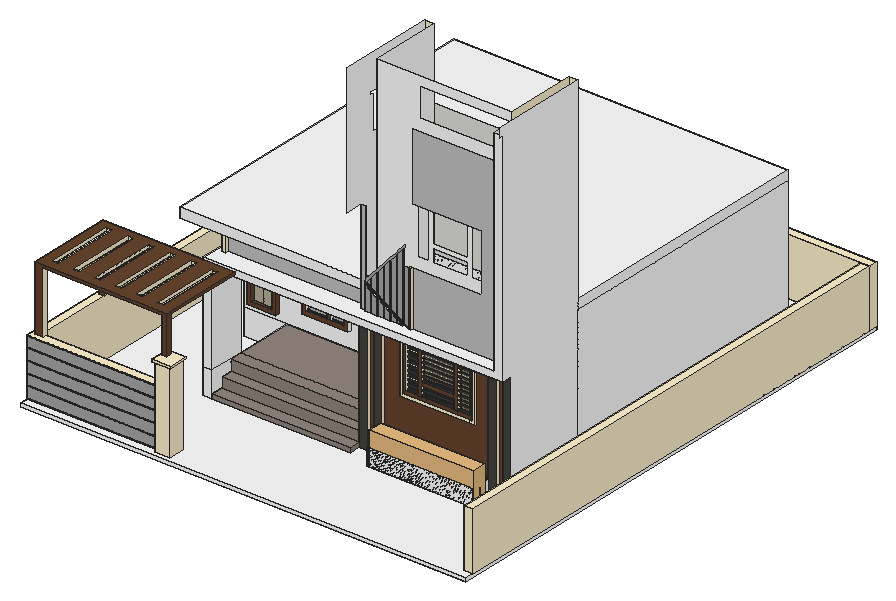
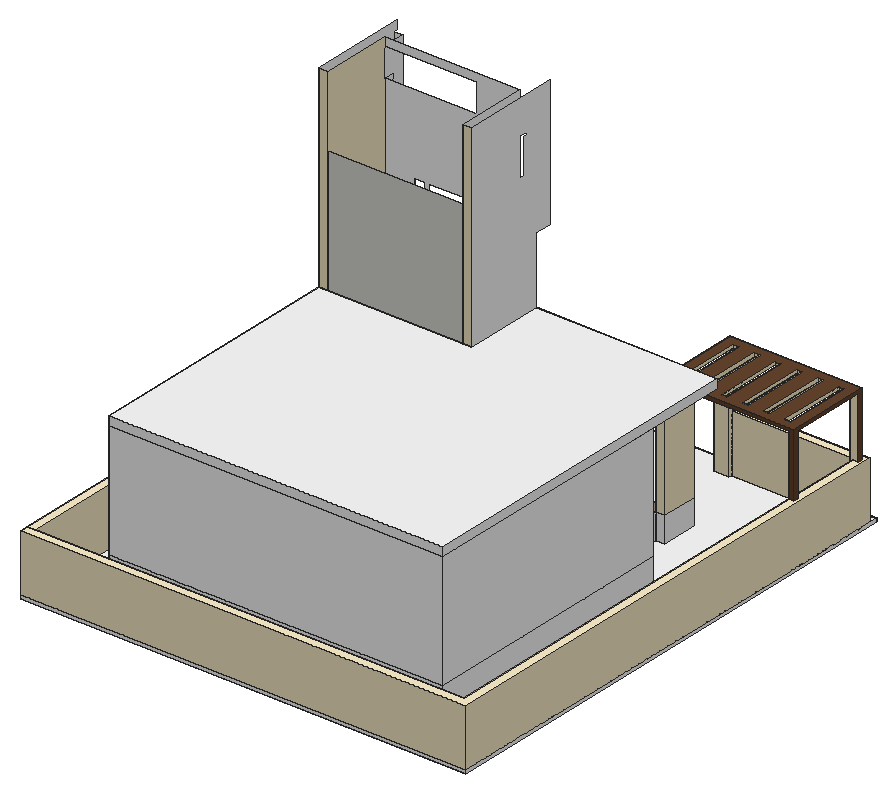
# SketchUp Ruby script. Lengths in inches.
U = 1.inch
M = Sketchup.active_model
def pt(a) = Geom::Point3d.new(a.map { |v| v * U })
def face(e, loops, mat)
  f = e.add_face(loops[0].map { |a| pt(a) })
  loops[1..].each { |l| e.add_face(l.map { |a| pt(a) }).erase! }
  f.material = f.back_material = mat if mat
  f
end
# faces: each face lists its corners as indices into pts; further lists are holes
def faces(e, pts, list, mat = nil) = list.each { |f| face(e, (f[0].is_a?(Array) ? f : [f]).map { |l| l.map { |i| pts[i] } }, mat) }
# xy, xz, yz: faces in a plane at the given z, y or x. An outline is a flat list of corners, or four numbers for a rectangle; further outlines are holes
def ring(l) = l.size == 4 ? [[l[0], l[1]], [l[2], l[1]], [l[2], l[3]], [l[0], l[3]]] : l.each_slice(2).to_a
def flat(e, list, mat, &to3) = list.each { |f| face(e, (f[0].is_a?(Array) ? f : [f]).map { |l| ring(l).map { |u, v| to3.(u, v) } }, mat) }
def xy(e, z, list, mat = nil) = flat(e, list, mat) { |x, y| [x, y, z] }
def xz(e, y, list, mat = nil) = flat(e, list, mat) { |x, z| [x, y, z] }
def yz(e, x, list, mat = nil) = flat(e, list, mat) { |y, z| [x, y, z] }
def lines(e, pts, list) = list.each { |a, b| e.add_line(pt(pts[a]), pt(pts[b])) }
# prism: a flat outline (further loops are holes) pulled along v
def prism(e, loops, v, mat = nil)
  f = face(e, loops, mat); d = Geom::Vector3d.new(v.map { |x| x * U })
  f.pushpull(f.normal.samedirection?(d) ? d.length : -d.length)
end
def box(e, o, s, mat = nil) = prism(e, [[o, [o[0] + s[0], o[1], o[2]], [o[0] + s[0], o[1] + s[1], o[2]], [o[0], o[1] + s[1], o[2]]]], [0, 0, s[2]], mat)
def at(x, y, z, deg = 0) = Geom::Transformation.translation(pt([x, y, z])) * Geom::Transformation.rotation(ORIGIN, Z_AXIS, deg.degrees)
def axes(o, x, y, z) = Geom::Transformation.new([*x, 0, *y, 0, *z, 0, *pt(o).to_a, 1])
def part(name) = M.definitions.add(name)
# library, detail: a bought-in or finely detailed component or shape, given as its bounding box
def library(name, o, s) = part(name).tap { |d| box(d.entities, o, s) }
def detail(e, o, s) = box(e.add_group.entities, o, s)
def put(e, d, t, mat = nil) = e.add_instance(d, t).tap { |i| i.material = mat if mat }
def group(e, t, mat = nil) = e.add_group.tap { |g| g.transformation = t; g.material = mat if mat }.entities
root = M.entities
M.materials.add("ARMANI GRIS").color = [147, 135, 128]
M.materials.add("D01_Frost_White").color = [255, 242, 206]
M.materials.add("Glass_Mirror_01").color = [255, 239, 176]
M.materials["Glass_Mirror_01"].alpha = 0.4
M.materials.add("Glass_Mirror_1").color = [185, 176, 151]
M.materials.add("Glass_Mirror_2").color = [185, 185, 185]
M.materials.add("M00_Soft_Cloud").color = [255, 255, 255]
M.materials.add("M02_Ash_Whisper").color = [196, 196, 196]
M.materials.add("M03_Pewter_Shine").color = [168, 168, 168]
M.materials.add("Metal_06_1K").color = [238, 236, 219]
M.materials.add("Wood_Planks_01_1K").color = [69, 67, 63]
M.materials.add("Wood_Veneer_15_1K").color = [103, 69, 45]
c1 = library("Planted timber trough",[0,0,0],[56.02,15.3,25.28])
box(root,[165.21,198.875,68.27],[13.86,1.29,0.92])
box(root,[139.02,198.6,107.3125],[40,1.1,0.73])
xy(root,0.86,[[396.02,114,405.02,117]],"D01_Frost_White")
xy(root,3.35,[[136.375,5.07,151.98,21.62],[0,9,0,534.44,464.04,534.44,464.04,525.44,9,525.44,9,18,136.375,18,136.375,9],[455.04,9,464.04,525.44],[411.02,114,411.02,117,285.02,117,285.02,115,276.02,115,276.02,117,270.02,117,270.02,115,261.02,115,261.02,201,270.02,201,270.02,126,411.02,126,411.02,201,420.02,201,420.02,114],[72.02,201,420.02,474.44]],"D01_Frost_White")
xy(root,30,[[270.02,126,411.02,201],[72.02,201,420.02,474.44]],"D01_Frost_White")
xy(root,52.05,[[139.02,198.6,179.02,199.7]])
xy(root,52.78,[[139.02,198.6,179.02,199.7]])
xy(root,57.57,[[139.02,198.6,179.02,199.7]])
xy(root,58.3,[[139.02,198.6,179.02,199.7]])
xy(root,61.28,[[3.55,14.22,3.55,18,9,18,9,19.37,12.18,19.37,12.18,14.22]],"D01_Frost_White")
xy(root,63.1,[[139.02,198.6,179.02,199.7]])
xy(root,63.35,[[0,9,136.375,9,136.375,18,3.55,18,3.55,19.37,9,19.37,9,98.26,3.55,98.26,3.55,103.1,9,103.1,9,525.44,464.04,525.44,464.04,534.44,0,534.44],[455.04,9,464.04,525.44],[3.55,18,9,19.37],[3.55,98.26,9,103.1]],"D01_Frost_White")
xy(root,63.83,[[139.02,198.6,179.02,199.7]])
xy(root,66,[[303.02,115,381.02,117]],"D01_Frost_White")
xy(root,68.625,[[139.02,198.6,142.56,199.7]])
xy(root,69,[[306.02,115,378.02,115.91]],"D01_Frost_White")
xy(root,69.35,[[139.02,198.6,142.56,199.7]])
xy(root,72,[[309.02,115.91,321.02,120.95],[325.02,115.91,359.02,120.95],[363.02,115.91,375.02,120.95],[309.02,120.95,321.02,126],[325.02,120.95,359.02,126],
  [363.02,120.95,375.02,126]],"D01_Frost_White")
xy(root,73.52,[[308.09,116.31,375.02,118.33]],"Wood_Planks_01_1K")
xy(root,74.15,[[139.02,198.6,179.02,199.7]])
xy(root,74.88,[[139.02,198.6,179.02,199.7]])
xy(root,74.89,[[308.09,116.31,375.02,118.33]],"Wood_Planks_01_1K")
xy(root,77.86,[[308.09,116.31,375.02,118.33]],"Wood_Planks_01_1K")
xy(root,79.23,[[308.09,116.31,375.02,118.33]],"Wood_Planks_01_1K")
xy(root,79.68,[[139.02,198.6,179.02,199.7]])
xy(root,80.41,[[139.02,198.6,179.02,199.7]])
xy(root,82.2,[[308.09,116.31,375.02,118.33]],"Wood_Planks_01_1K")
xy(root,82.48,[[325.02,115.91,359.02,120.95],[325.02,120.95,359.02,126]],"D01_Frost_White")
xy(root,83.57,[[308.09,116.31,375.02,118.33]],"Wood_Planks_01_1K")
xy(root,85.21,[[139.02,198.6,179.02,199.7]])
xy(root,85.93,[[139.02,198.6,179.02,199.7]])
xy(root,86.1,[[136.32,14.22,140.85,19.37]],"D01_Frost_White")
xy(root,86.48,[[325.02,115.91,359.02,120.95],[325.02,120.95,359.02,126]],"D01_Frost_White")
xy(root,86.54,[[308.09,116.31,375.02,118.33]],"Wood_Planks_01_1K")
xy(root,87.91,[[308.09,116.31,375.02,118.33]],"Wood_Planks_01_1K")
xy(root,88.07,[[134.375,3.07,153.98,5.07],[134.375,5.07,136.375,23.62],[136.375,5.07,151.98,21.62],[151.98,5.07,153.98,23.62],[136.375,21.62,151.98,23.62]],"D01_Frost_White")
xy(root,90.29,[[134.375,3.07,153.98,23.62]],"D01_Frost_White")
xy(root,90.73,[[139.02,198.6,179.02,199.7]])
xy(root,90.88,[[308.09,116.31,375.02,118.33]],"Wood_Planks_01_1K")
xy(root,91.46,[[139.02,198.6,179.02,199.7]])
xy(root,92.25,[[308.09,116.31,375.02,118.33]],"Wood_Planks_01_1K")
xy(root,95.22,[[308.09,116.31,375.02,118.33]],"Wood_Planks_01_1K")
xy(root,96.26,[[139.02,198.6,179.02,199.7]])
xy(root,96.59,[[308.09,116.31,375.02,118.33]],"Wood_Planks_01_1K")
xy(root,96.99,[[139.02,198.6,179.02,199.7]])
xy(root,99.5625,[[308.09,116.31,375.02,118.33]],"Wood_Planks_01_1K")
xy(root,100.93,[[308.09,116.31,375.02,118.33]],"Wood_Planks_01_1K")
xy(root,101.79,[[139.02,198.6,179.02,199.7]])
xy(root,102.51,[[139.02,198.6,179.02,199.7]])
xy(root,103.9,[[308.09,116.31,375.02,118.33]],"Wood_Planks_01_1K")
xy(root,105.27,[[308.09,116.31,375.02,118.33]],"Wood_Planks_01_1K")
xy(root,108.24,[[308.09,116.31,375.02,118.33]],"Wood_Planks_01_1K")
xy(root,109.61,[[308.09,116.31,375.02,118.33]],"Wood_Planks_01_1K")
xy(root,112.58,[[308.09,116.31,375.02,118.33]],"Wood_Planks_01_1K")
xy(root,113.95,[[308.09,116.31,375.02,118.33]],"Wood_Planks_01_1K")
xy(root,116.92,[[308.09,116.31,375.02,118.33]],"Wood_Planks_01_1K")
xy(root,118.29,[[308.09,116.31,375.02,118.33]],"Wood_Planks_01_1K")
xy(root,120,[[309.02,115.91,321.02,120.95],[325.02,115.91,359.02,120.95],[363.02,115.91,375.02,120.95],[309.02,120.95,321.02,126],[325.02,120.95,359.02,126],
  [363.02,120.95,375.02,126]],"D01_Frost_White")
xy(root,123,[[306.02,115,378.02,115.91]],"D01_Frost_White")
xy(root,125.52,[[117.02,103.1,117.02,115,381.02,115,381.02,117,396.02,117,396.02,114,405.02,114,405.02,117,411.02,117,411.02,103.1],[117.02,115,261.02,140.4],[270.02,115,276.02,117],[285.02,115,303.02,117]],"D01_Frost_White")
xy(root,126,[[303.02,115,381.02,117]],"D01_Frost_White")
xy(root,127.21,[[12.18,14.22,136.32,19.37],[[3.55,19.37,3.55,98.26,9,98.26,9,103.1,140.85,103.1,140.85,19.37],[124.16,24.36,129.84,94.44],[102.125,24.36,107.8,94.44],[80.09,24.36,85.76,94.44],[58.05,24.36,63.72,94.44],[36.01,24.36,41.68,94.44],[13.97,24.36,19.65,94.44]]],"Wood_Veneer_15_1K")
xy(root,130.28,[[[3.55,14.22,140.85,103.1],[13.97,24.36,19.65,94.44],[36.01,24.36,41.68,94.44],[58.05,24.36,63.72,94.44],[80.09,24.36,85.76,94.44],[102.125,24.36,107.8,94.44],[124.16,24.36,129.84,94.44]]],"Wood_Veneer_15_1K")
xy(root,132.15,[[117.48,123.86,261.02,140.4],[113.03,129.7,117.48,140.4],[113.03,140.4,117.48,141.42],[113.03,141.42,117.48,201]],"D01_Frost_White")
xy(root,132.15,[[108.02,103.1,411.02,103.1,411.02,117,315.02,117,315.02,115,313.02,115,313.02,117,312.52,117,312.52,116,310.92,116,310.92,117,305.81,117,305.81,116,299.59,116,299.59,117,299.09,117,299.09,116,292.88,116,292.88,117,292.38,117,292.38,116,286.17,116,286.17,117,285.67,117,285.67,116,279.45,116,279.45,117,278.95,117,278.95,116,272.74,116,272.74,117,272.24,117,272.24,116,266.02,116,266.02,117,261.02,117,261.02,123.86,117.48,123.86,117.48,120.75,113.03,120.75,113.03,140.4,108.02,140.4]],"M00_Soft_Cloud")
xy(root,134.89,[[113.03,126.97,115.26,129.7],[115.26,126.97,117.48,129.7],[113.03,129.7,115.26,141.42],[115.26,129.7,117.48,141.42],[113.03,141.42,115.26,201],
  [115.26,141.42,117.48,201]],"D01_Frost_White")
xy(root,150.59,[[113.03,120.75,117.48,126.97]],"D01_Frost_White")
xz(root,3.07,[[134.375,88.07,153.98,90.29]],"D01_Frost_White")
xz(root,5.07,[[136.375,3.35,151.98,88.07]],"D01_Frost_White")
xz(root,9,[[0,3.35,136.375,4.35],[455.04,3.35,464.04,63.35],[0,15.15,136.375,16.15],[0,26.95,136.375,27.95],[0,38.75,136.375,39.75],
  [0,50.55,136.375,51.55],[0,62.35,136.375,63.35]],"D01_Frost_White")
xz(root,9,[[0,4.35,136.375,15.15],[0,16.15,136.375,26.95],[0,27.95,136.375,38.75],[0,39.75,136.375,50.55],[0,51.55,136.375,62.35]],"M03_Pewter_Shine")
xz(root,14.22,[[3.55,61.28,12.18,61.28,12.18,127.21,136.32,127.21,136.32,86.1,140.85,86.1,140.85,130.28,3.55,130.28]],"Wood_Veneer_15_1K")
xz(root,18,[[9,3.35,136.375,63.35],[3.55,61.28,9,63.35]],"D01_Frost_White")
xz(root,19.37,[[9,61.28,9,63.35,3.55,63.35,3.55,127.21,12.18,127.21,12.18,61.28],[136.32,86.1,140.85,127.21]],"D01_Frost_White")
xz(root,21.62,[[136.375,3.35,151.98,88.07]],"D01_Frost_White")
xz(root,23.62,[[134.375,88.07,153.98,90.29]],"D01_Frost_White")
xz(root,24.36,[[13.97,127.21,19.65,130.28],[36.01,127.21,41.68,130.28],[58.05,127.21,63.72,130.28],[80.09,127.21,85.76,130.28],[102.125,127.21,107.8,130.28],
  [124.16,127.21,129.84,130.28]],"D01_Frost_White")
xz(root,94.44,[[13.97,127.21,19.65,130.28],[36.01,127.21,41.68,130.28],[58.05,127.21,63.72,130.28],[80.09,127.21,85.76,130.28],[102.125,127.21,107.8,130.28],
  [124.16,127.21,129.84,130.28]],"D01_Frost_White")
xz(root,98.26,[[3.55,63.35,9,127.21]],"Wood_Veneer_15_1K")
xz(root,103.1,[[108.02,30,117.02,30,117.02,125.52,411.02,125.52,411.02,125.51,420.02,125.6,420.02,355,411.02,355,411.02,132.15,108.02,132.15,108.02,130.28,140.85,130.28,140.85,127.21,108.02,127.21]],"M00_Soft_Cloud")
xz(root,103.1,[[3.55,63.35,3.55,130.28,108.02,130.28,108.02,127.21,9,127.21,9,63.35]],"Wood_Veneer_15_1K")
xz(root,114,[[396.02,0.86,405.02,125.52],[411.02,3.35,420.02,3.35,420.02,125.6,411.02,125.51]],"Wood_Planks_01_1K")
xz(root,115,[[[303.02,66,381.02,125.52],[306.02,69,378.02,123]],[303.02,125.52,381.02,126],[313.02,132.15,315.02,188.68]],"D01_Frost_White")
xz(root,115,[[261.02,3.35,270.02,125.52],[276.02,3.35,285.02,125.52]],"Wood_Planks_01_1K")
xz(root,115.91,[[[306.02,69,378.02,123],[309.02,72,375.02,120]],[321.02,72,325.02,120],[359.02,72,363.02,120],[325.02,82.48,359.02,86.48]],"Wood_Veneer_15_1K")
xz(root,116,[[266.02,132.15,272.24,132.15,272.24,152.97,266.02,156.83],[272.74,132.15,278.95,132.15,278.95,148.81,272.74,152.66],[279.45,132.15,285.67,132.15,285.67,144.64,279.45,148.5],[286.17,132.15,292.38,132.15,292.38,140.48,286.17,144.33],[292.88,132.15,299.09,132.15,299.09,136.3125,292.88,140.17],
  [299.59,132.15,305.81,132.15,299.59,136],[310.92,132.15,312.52,132.15,312.52,188.68,307.01,188.68,307.01,204.4375,306.31,203.62,306.31,135.04],[305.81,135.35,305.81,203.04,299.59,195.82,299.59,139.26],[299.09,139.57,299.09,195.24,292.88,188.02,292.88,143.47],[292.38,143.78,292.38,187.44,286.17,180.22,286.17,147.68],
  [285.67,148,285.67,179.64,279.45,172.42,279.45,151.9],[278.95,152.21,278.95,171.84,272.74,164.625,272.74,156.11],[272.24,156.43,272.24,164.05,267.98,159.1]],"M03_Pewter_Shine")
xz(root,116.31,[[308.09,73.52,375.02,74.89],[308.09,77.86,375.02,79.23],[308.09,82.2,375.02,83.57],[308.09,86.54,375.02,87.91],[308.09,90.88,375.02,92.25],
  [308.09,95.22,375.02,96.59],[308.09,99.5625,375.02,100.93],[308.09,103.9,375.02,105.27],[308.09,108.24,375.02,109.61],[308.09,112.58,375.02,113.95],
  [308.09,116.92,375.02,118.29]],"Wood_Planks_01_1K")
xz(root,117,[[396.02,0.86,405.02,3.35],[265.52,132.15,266.02,229.42],[272.24,132.15,272.74,132.15,272.74,152.66,272.24,152.97],[278.95,132.15,279.45,132.15,279.45,148.5,278.95,148.81],[285.67,132.15,286.17,132.15,286.17,144.33,285.67,144.64],
  [292.38,132.15,292.88,132.15,292.88,140.17,292.38,140.48],[299.09,132.15,299.59,132.15,299.59,136,299.09,136.3125],[312.52,132.15,313.02,188.68],[306.31,135.04,306.31,203.62,305.81,203.04,305.81,135.35],[299.59,139.26,299.59,195.82,299.09,195.24,299.09,139.57],
  [292.88,143.47,292.88,188.02,292.38,187.44,292.38,143.78],[286.17,147.68,286.17,180.22,285.67,179.64,285.67,148],[279.45,151.9,279.45,172.42,278.95,171.84,278.95,152.21],[272.74,156.11,272.74,164.625,272.24,164.05,272.24,156.43]],"D01_Frost_White")
xz(root,117,[[261.02,132.15,265.52,132.15,265.52,157.14,263.68,158.28,265.52,160.37,265.52,229.42,261.02,229.42],[315.02,132.15,411.02,132.15,411.02,319,315.02,319,315.02,248.68,387.02,248.68,387.02,188.68,315.02,188.68]],"M02_Ash_Whisper")
xz(root,117,[[305.81,132.15,310.92,132.15,306.31,135.04,305.81,135.35,299.59,139.26,299.09,139.57,292.88,143.47,292.38,143.78,286.17,147.68,285.67,148,279.45,151.9,278.95,152.21,272.74,156.11,272.24,156.43,267.98,159.1,272.24,164.05,272.74,164.625,278.95,171.84,279.45,172.42,285.67,179.64,286.17,180.22,292.38,187.44,292.88,188.02,299.09,195.24,299.59,195.82,305.81,203.04,306.31,203.62,307.01,204.4375,307.01,207.4375,306.31,206.64,305.81,206.07,299.59,199.02,299.09,198.46,292.88,191.4,292.38,190.84,286.17,183.79,285.67,183.22,279.45,176.17,278.95,175.6,272.74,168.55,272.24,167.99,266.02,160.9375,266.02,156.83,272.24,152.97,272.74,152.66,278.95,148.81,279.45,148.5,285.67,144.64,286.17,144.33,292.38,140.48,292.88,140.17,299.09,136.3125,299.59,136],[265.52,157.14,265.52,160.37,263.68,158.28]],"M03_Pewter_Shine")
xz(root,117,[[270.02,3.35,276.02,125.52],[285.02,3.35,396.02,3.35,396.02,125.52,381.02,125.52,381.02,66,303.02,66,303.02,125.52,285.02,125.52],[405.02,3.35,411.02,125.52]],"Wood_Veneer_15_1K")
xz(root,118.33,[[308.09,73.52,375.02,74.89],[308.09,77.86,375.02,79.23],[308.09,82.2,375.02,83.57],[308.09,86.54,375.02,87.91],[308.09,90.88,375.02,92.25],
  [308.09,95.22,375.02,96.59],[308.09,99.5625,375.02,100.93],[308.09,103.9,375.02,105.27],[308.09,108.24,375.02,109.61],[308.09,112.58,375.02,113.95],
  [308.09,116.92,375.02,118.29]],"Wood_Planks_01_1K")
xz(root,120.75,[[113.03,132.15,117.48,150.59]],"D01_Frost_White")
xz(root,120.95,[[309.02,72,321.02,120],[325.02,72,359.02,82.48]],"D01_Frost_White")
xz(root,120.95,[[363.02,72,375.02,120],[325.02,86.48,359.02,120]],"Glass_Mirror_01")
xz(root,123.86,[[117.48,132.15,261.02,150]],"M02_Ash_Whisper")
xz(root,126,[[270.02,3.35,411.02,30]],"D01_Frost_White")
xz(root,126,[[[270.02,30,270.02,364,411.02,364,411.02,355,315.02,355,315.02,325,411.02,325,411.02,30],[325.02,86.48,359.02,120],[329.01,212.1,365.01,242.68],[369.01,194.68,381.02,242.68],[363.02,72,375.02,120],[313.01,194.68,325.01,242.68],[309.02,72,321.02,120],[329.01,194.68,365.01,208.1],[325.02,72,359.02,82.48]]],"M00_Soft_Cloud")
xz(root,126.97,[[113.03,134.89,117.48,150.59]],"D01_Frost_White")
xz(root,129.7,[[113.03,132.15,117.48,134.89]],"D01_Frost_White")
xz(root,140.4,[[108.02,30,108.02,132.15,261.02,132.15,261.02,125.52,117.02,125.52,117.02,30]],"D01_Frost_White")
xz(root,141.42,[[113.03,132.15,117.48,134.89]],"D01_Frost_White")
xz(root,198.6,[[139.02,52.05,179.02,52.78],[139.02,57.57,179.02,58.3],[139.02,63.1,179.02,63.83],[139.02,68.625,142.56,69.35],[139.02,74.15,179.02,74.88],
  [139.02,79.68,179.02,80.41],[139.02,85.21,179.02,85.93],[139.02,90.73,179.02,91.46],[139.02,96.26,179.02,96.99],[139.02,101.79,179.02,102.51]])
xz(root,199.7,[[139.02,52.05,179.02,52.78],[139.02,57.57,179.02,58.3],[139.02,63.1,179.02,63.83],[139.02,68.625,142.56,69.35],[139.02,74.15,179.02,74.88],
  [139.02,79.68,179.02,80.41],[139.02,85.21,179.02,85.93],[139.02,90.73,179.02,91.46],[139.02,96.26,179.02,96.99],[139.02,101.79,179.02,102.51]])
xz(root,201,[[270.02,30,411.02,290]])
xz(root,201,[[261.02,3.35,270.02,30],[270.02,3.35,411.02,30],[411.02,3.35,420.02,30],[261.02,30,270.02,364],[411.02,30,420.02,364],
  [113.03,132.15,117.48,134.89]],"D01_Frost_White")
xz(root,201,[[72.02,3.35,261.02,30]],"M00_Soft_Cloud")
xz(root,474.44,[[72.02,3.35,420.02,30]],"M00_Soft_Cloud")
xz(root,525.44,[[9,3.35,455.04,63.35],[455.04,3.35,464.04,63.35]],"D01_Frost_White")
xz(root,534.44,[[0,3.35,464.04,63.35]],"D01_Frost_White")
yz(root,0,[[9,3.35,534.44,63.35]],"D01_Frost_White")
yz(root,3.55,[[14.22,61.28,14.22,130.28,103.1,130.28,103.1,63.35,98.26,63.35,98.26,127.21,19.37,127.21,19.37,63.35,18,63.35,18,61.28]],"Wood_Veneer_15_1K")
yz(root,9,[[18,3.35,525.44,3.35,525.44,63.35,19.37,63.35,19.37,61.28,18,61.28],[18,61.28,19.37,63.35],[98.26,63.35,103.1,127.21]],"D01_Frost_White")
yz(root,12.18,[[14.22,61.28,19.37,127.21]],"D01_Frost_White")
yz(root,13.97,[[24.36,127.21,94.44,130.28]],"D01_Frost_White")
yz(root,19.65,[[24.36,127.21,94.44,130.28]],"D01_Frost_White")
yz(root,36.01,[[24.36,127.21,94.44,130.28]],"D01_Frost_White")
yz(root,41.68,[[24.36,127.21,94.44,130.28]],"D01_Frost_White")
yz(root,58.05,[[24.36,127.21,94.44,130.28]],"D01_Frost_White")
yz(root,63.72,[[24.36,127.21,94.44,130.28]],"D01_Frost_White")
yz(root,72.02,[[201,3.35,474.44,30]],"M00_Soft_Cloud")
yz(root,80.09,[[24.36,127.21,94.44,130.28]],"D01_Frost_White")
yz(root,85.76,[[24.36,127.21,94.44,130.28]],"D01_Frost_White")
yz(root,102.125,[[24.36,127.21,94.44,130.28]],"D01_Frost_White")
yz(root,107.8,[[24.36,127.21,94.44,130.28]],"D01_Frost_White")
yz(root,108.02,[[103.1,30,140.4,132.15]],"D01_Frost_White")
yz(root,113.03,[[120.75,132.15,120.75,150.59,126.97,150.59,126.97,134.89,129.7,134.89,129.7,132.15],[129.7,132.15,141.42,134.89],[141.42,132.15,201,134.89]],"D01_Frost_White")
yz(root,115.26,[[126.97,134.89,201,150]],"M03_Pewter_Shine")
yz(root,117.02,[[103.1,30,140.4,125.52]],"M00_Soft_Cloud")
yz(root,117.48,[[120.75,132.15,129.7,132.15,129.7,134.89,126.97,134.89,126.97,150.59,120.75,150.59],[129.7,132.15,141.42,134.89],[141.42,132.15,201,134.89]],"D01_Frost_White")
yz(root,124.16,[[24.36,127.21,94.44,130.28]],"D01_Frost_White")
yz(root,129.84,[[24.36,127.21,94.44,130.28]],"D01_Frost_White")
yz(root,134.375,[[3.07,88.07,23.62,90.29]],"D01_Frost_White")
yz(root,136.32,[[14.22,86.1,19.37,127.21]],"Wood_Veneer_15_1K")
yz(root,136.375,[[5.07,3.35,5.07,88.07,21.62,88.07,21.62,3.35,18,3.35,18,63.35,9,63.35,9,3.35],[9,3.35,18,63.35]],"D01_Frost_White")
yz(root,140.85,[[14.22,86.1,19.37,86.1,19.37,127.21,103.1,127.21,103.1,130.28,14.22,130.28]],"Wood_Veneer_15_1K")
yz(root,142.56,[[198.6,68.625,199.7,69.35]])
yz(root,151.98,[[5.07,3.35,21.62,88.07]],"D01_Frost_White")
yz(root,153.98,[[3.07,88.07,23.62,90.29]],"D01_Frost_White")
yz(root,179.02,[[198.6,52.05,199.7,52.78],[198.6,57.57,199.7,58.3],[198.6,63.1,199.7,63.83],[198.6,74.15,199.7,74.88],[198.6,79.68,199.7,80.41],
  [198.6,85.21,199.7,85.93],[198.6,90.73,199.7,91.46],[198.6,96.26,199.7,96.99],[198.6,101.79,199.7,102.51]])
yz(root,261.02,[[[115,3.35,115,125.52,140.4,125.52,140.4,132.15,117,132.15,117,229.42,99,229.42,99,364,201,364,201,3.35],[133.24,290,138,290,138,328.95,129,328.95,129,326,132.24,326,132.24,320,133.24,320,133.24,319,132.24,319,132.24,312.75,133.24,312.75,133.24,311.75,132.24,311.75,132.24,305.5,133.24,305.5,133.24,304.5,132.24,304.5,132.24,298.25,133.24,298.25,133.24,297.25,132.24,297.25,132.24,291,133.24,291]]],"M00_Soft_Cloud")
yz(root,266.02,[[116,132.15,117,156.83]],"D01_Frost_White")
yz(root,270.02,[[115,3.35,117,125.52],[126,3.35,201,30]],"D01_Frost_White")
yz(root,270.02,[[126,30,201,364]],"M00_Soft_Cloud")
yz(root,272.24,[[116,132.15,117,152.97],[116,156.43,117,164.05]],"D01_Frost_White")
yz(root,272.74,[[116,132.15,117,152.66],[116,156.11,117,164.625]],"D01_Frost_White")
yz(root,276.02,[[115,3.35,117,125.52]],"D01_Frost_White")
yz(root,278.95,[[116,132.15,117,148.81],[116,152.21,117,171.84]],"D01_Frost_White")
yz(root,279.45,[[116,132.15,117,148.5],[116,151.9,117,172.42]],"D01_Frost_White")
yz(root,285.02,[[115,3.35,117,125.52]],"D01_Frost_White")
yz(root,285.67,[[116,132.15,117,144.64],[116,148,117,179.64]],"D01_Frost_White")
yz(root,286.17,[[116,132.15,117,144.33],[116,147.68,117,180.22]],"D01_Frost_White")
yz(root,292.38,[[116,132.15,117,140.48],[116,143.78,117,187.44]],"D01_Frost_White")
yz(root,292.88,[[116,132.15,117,140.17],[116,143.47,117,188.02]],"D01_Frost_White")
yz(root,299.09,[[116,132.15,117,136.3125],[116,139.57,117,195.24]],"D01_Frost_White")
yz(root,299.59,[[116,132.15,117,136],[116,139.26,117,195.82]],"D01_Frost_White")
yz(root,303.02,[[115,66,117,125.52],[115,125.52,117,126]],"D01_Frost_White")
yz(root,305.81,[[116,135.35,117,203.04]],"D01_Frost_White")
yz(root,306.02,[[115,69,115.91,123]],"D01_Frost_White")
yz(root,306.31,[[116,135.04,117,203.62]],"D01_Frost_White")
yz(root,309.02,[[115.91,72,120.95,120],[120.95,72,126,120]],"D01_Frost_White")
yz(root,312.52,[[116,132.15,117,188.68]],"D01_Frost_White")
yz(root,313.02,[[115,132.15,117,188.68]],"D01_Frost_White")
yz(root,315.02,[[115,132.15,117,188.68]],"D01_Frost_White")
yz(root,321.02,[[115.91,72,120.95,120],[120.95,72,126,120]],"D01_Frost_White")
yz(root,325.02,[[115.91,72,120.95,82.48],[120.95,72,126,82.48],[115.91,86.48,120.95,120],[120.95,86.48,126,120]],"D01_Frost_White")
yz(root,359.02,[[115.91,72,120.95,82.48],[120.95,72,126,82.48],[115.91,86.48,120.95,120],[120.95,86.48,126,120]],"D01_Frost_White")
yz(root,363.02,[[115.91,72,120.95,120],[120.95,72,126,120]],"D01_Frost_White")
yz(root,375.02,[[[115.91,72,120.95,120],[116.31,99.5625,118.33,100.93],[116.31,90.88,118.33,92.25],[116.31,86.54,118.33,87.91],[116.31,82.2,118.33,83.57],[116.31,77.86,118.33,79.23],[116.31,73.52,118.33,74.89],[116.31,95.22,118.33,96.59],[116.31,103.9,118.33,105.27],[116.31,108.24,118.33,109.61],[116.31,112.58,118.33,113.95],[116.31,116.92,118.33,118.29]],[120.95,72,126,120]],"D01_Frost_White")
yz(root,378.02,[[115,69,115.91,123]],"D01_Frost_White")
yz(root,381.02,[[115,66,117,125.52],[115,125.52,117,126]],"D01_Frost_White")
yz(root,396.02,[[114,0.86,117,125.51],[114,125.51,117,125.52]],"D01_Frost_White")
yz(root,405.02,[[114,0.86,117,125.51],[114,125.51,117,125.52]],"D01_Frost_White")
yz(root,411.02,[[114,3.35,117,125.51],[126,3.35,201,30],[126,30,201,364],[103.1,125.51,117,125.52]],"D01_Frost_White")
yz(root,411.02,[[103.1,132.15,103.1,355,126,355,126,325,114,325,114,319,117,319,117,132.15]],"M00_Soft_Cloud")
yz(root,420.02,[[114,3.35,201,3.35,201,364,99,364,99,355,103.1,355,103.1,125.6,114,125.6],[201,3.35,474.44,30]],"M00_Soft_Cloud")
yz(root,455.04,[[9,3.35,525.44,63.35]],"D01_Frost_White")
yz(root,464.04,[[9,3.35,525.44,63.35],[525.44,3.35,534.44,63.35]],"D01_Frost_White")
p = [[420.02,114,125.6],[420.02,103.1,125.6],[411.02,103.1,125.51],[411.02,114,125.51],[299.59,116,136],[305.81,116,132.15],
  [305.81,117,132.15],[299.59,117,136],[310.92,116,132.15],[306.31,116,135.04],[306.31,117,135.04],[310.92,117,132.15],
  [305.81,116,135.35],[299.59,116,139.26],[299.59,117,139.26],[305.81,117,135.35],[292.88,116,140.17],[299.09,116,136.3125],
  [299.09,117,136.3125],[292.88,117,140.17],[299.09,116,139.57],[292.88,116,143.47],[292.88,117,143.47],[299.09,117,139.57],
  [286.17,116,144.33],[292.38,116,140.48],[292.38,117,140.48],[286.17,117,144.33],[292.38,116,143.78],[286.17,116,147.68],
  [286.17,117,147.68],[292.38,117,143.78],[279.45,116,148.5],[285.67,116,144.64],[285.67,117,144.64],[279.45,117,148.5],
  [285.67,116,148],[279.45,116,151.9],[279.45,117,151.9],[285.67,117,148],[272.74,116,152.66],[278.95,116,148.81],
  [278.95,117,148.81],[272.74,117,152.66],[278.95,116,152.21],[272.74,116,156.11],[272.74,117,156.11],[278.95,117,152.21],
  [266.02,116,156.83],[272.24,116,152.97],[272.24,117,152.97],[266.02,117,156.83],[272.24,116,156.43],[267.98,116,159.1],
  [267.98,117,159.1],[272.24,117,156.43],[411.02,117,125.52],[411.02,117,125.6],[405.02,117,125.52],[405.02,117,125.6],
  [396.02,117,125.52],[396.02,117,125.6]]
faces(root,p,[[0,1,2,3]],"D01_Frost_White")
faces(root,p,[[4,5,6,7],[8,9,10,11],[12,13,14,15],[16,17,18,19],[20,21,22,23],[24,25,26,27],[28,29,30,31],[32,33,34,35],
  [36,37,38,39],[40,41,42,43],[44,45,46,47],[48,49,50,51],[52,53,54,55]],"Metal_06_1K")
lines(root,p,[[56,57],[58,59],[60,61]])
g1 = group(root,at(63.02,0,0),"M00_Soft_Cloud")
xy(g1,0,[[-63.02,0,401.02,534.44]])
xy(g1,3.35,[[[-63.02,0,401.02,534.44],[45,103.1,45,140.4,54,140.4,54,201,198,201,198,115,198.28,103.1],[222,94.6,222,117,333,117,333,114,333.29,103.1,333.29,94.6]]])
xy(g1,3.76,[[222.9375,95.54,332.35,95.54,332.35,103.09,332.0625,113.99,332.0625,116.0625,222.9375,116.0625]])
xy(g1,7.9,[[54,103.1,198.28,103.1,198,115,198,115.53,54,115.53]],"ARMANI GRIS")
xy(g1,18,[[54,115.53,198,127.97]],"ARMANI GRIS")
xy(g1,20.95,[[[222,94.6,333.29,94.6,333.29,103.1,333,114,333,117,222,117],[222.9375,95.54,222.9375,116.0625,332.0625,116.0625,332.0625,113.99,332.35,103.09,332.35,95.54]]])
xy(g1,30,[[54,127.97,198,140.4],[54,140.4,198,201]],"ARMANI GRIS")
xz(g1,0,[[-63.02,0,401.02,3.35]])
xz(g1,94.6,[[222,3.35,333.29,20.95]])
xz(g1,95.54,[[222.9375,3.76,332.35,20.95]])
xz(g1,103.1,[[45,3.35,54,30]])
xz(g1,103.1,[[54,3.35,198.28,7.9]],"ARMANI GRIS")
xz(g1,115.53,[[54,7.9,198,18]],"ARMANI GRIS")
xz(g1,116.0625,[[222.9375,3.76,332.0625,20.95]])
xz(g1,117,[[222,3.35,333,20.95]])
xz(g1,127.97,[[54,18,198,30]],"ARMANI GRIS")
xz(g1,140.4,[[45,3.35,54,30]])
xz(g1,201,[[54,3.35,198,30]])
xz(g1,534.44,[[-63.02,0,401.02,3.35]])
yz(g1,-63.02,[[0,0,534.44,3.35]])
yz(g1,45,[[103.1,3.35,140.4,30]])
yz(g1,54,[[103.1,3.35,115.53,7.9],[115.53,3.35,127.97,18],[127.97,3.35,140.4,30],[140.4,3.35,201,30],[103.1,7.9,115.53,7.9,115.53,18,127.97,18,127.97,30,103.1,30]])
yz(g1,198,[[115,3.35,115.53,7.9],[115.53,3.35,127.97,18],[127.97,3.35,140.4,30],[140.4,3.35,201,30]])
yz(g1,222,[[94.6,3.35,115,20.95],[115,3.35,117,20.95]])
yz(g1,222.9375,[[95.54,3.76,115,20.95],[115,3.76,116.0625,20.95]])
yz(g1,332.0625,[[113.99,3.76,116.0625,20.95]])
yz(g1,332.35,[[95.54,3.76,103.09,20.95]])
yz(g1,333,[[114,3.35,117,20.95]])
yz(g1,333.29,[[94.6,3.35,103.1,20.95]])
yz(g1,401.02,[[0,0,534.44,3.35]])
p = [[198,115,3.35],[198,115,7.9],[198.28,103.1,7.9],[198.28,103.1,3.35],[333,114,20.95],[333.29,103.1,20.95],
  [333.29,103.1,3.35],[333,114,3.35],[332.35,103.09,20.95],[332.0625,113.99,20.95],[332.0625,113.99,3.76],[332.35,103.09,3.76],
  [198,201,30],[198.28,201,30],[198,115.53,30],[198.28,115.53,30],[198,127.97,30],[198.28,127.97,30],
  [198,140.4,30],[198.28,140.4,30]]
faces(g1,p,[[0,1,2,3]],"ARMANI GRIS")
faces(g1,p,[[4,5,6,7],[8,9,10,11]])
lines(g1,p,[[12,13],[14,15],[16,17],[18,19]])
put(root,c1,axes([287.49,94.6,3.76],[1.94267,0,0],[0,1,0],[0,0,1.3439]),"D01_Frost_White")
g2 = group(root,at(72.02,201,30),"M00_Soft_Cloud")
xy(g2,0,[[9,9,341.95,264.44]])
xy(g2,6,[[129,-3,177.21,0]])
xy(g2,6,[[5.93,-3,36,0]],"Wood_Veneer_15_1K")
xy(g2,10,[[133,-3,153.1,0],[157.1,-3,173.21,0]])
xy(g2,10,[[9.93,-3,32,0]],"Wood_Veneer_15_1K")
xy(g2,17.09,[[63,-3,111,0]])
xy(g2,21.09,[[67,-3,89.19,0],[93.19,-3,107,0]])
xy(g2,36.12,[[67,-3,89.19,0]])
xy(g2,40.12,[[67,-3,89.19,0]])
xy(g2,80,[[67,-3,89.19,0],[93.19,-3,107,0],[133,-3,153.1,0],[157.1,-3,173.21,0]])
xy(g2,84,[[63,-3,111,0],[129,-3,177.21,0]])
xy(g2,98,[[9.93,-3,32,0]])
xy(g2,102,[[5.93,-3,36,0]],"Wood_Veneer_15_1K")
xy(g2,120,[[[0,0,348,273.44],[9,9,341.95,264.44]]])
xz(g2,-3,[[[129,6,177.21,84],[133,10,173.21,80]],[153.1,10,157.1,80]],"Wood_Planks_01_1K")
xz(g2,-3,[[[5.93,6,36,102],[9.93,10,32,98]],[[63,17.09,111,84],[67,21.09,107,80]],[89.19,21.09,93.19,21.09,93.19,80,89.19,80,89.19,40.12,67,40.12,67,36.12,89.19,36.12]],"Wood_Veneer_15_1K")
xz(g2,0,[[[0,0,348,120],[129,6,177.21,84],[63,17.09,111,84],[5.93,6,36,102]]])
xz(g2,0,[[9.93,10,20.97,32],[20.97,10,32,32],[9.93,32,20.97,54],[20.97,32,32,54],[9.93,54,20.97,76],
  [20.97,54,32,76],[9.93,76,20.97,98],[20.97,76,32,98]],"Glass_Mirror_1")
xz(g2,0,[[67,21.09,89.19,36.12],[93.19,21.09,107,80],[67,40.12,89.19,80]],"Glass_Mirror_2")
xz(g2,0,[[133,10,153.1,80],[157.1,10,173.21,80]],"Wood_Veneer_15_1K")
xz(g2,9,[[9,0,341.95,120]])
xz(g2,264.44,[[9,0,341.95,120]])
xz(g2,273.44,[[0,0,348,120]])
yz(g2,0,[[0,0,273.44,120]])
yz(g2,5.93,[[-3,6,0,102]],"Wood_Veneer_15_1K")
yz(g2,9,[[9,0,264.44,120]])
yz(g2,9.93,[[-3,10,0,98]],"Wood_Veneer_15_1K")
yz(g2,32,[[-3,10,0,98]],"Wood_Veneer_15_1K")
yz(g2,36,[[-3,6,0,102]],"Wood_Veneer_15_1K")
yz(g2,63,[[-3,17.09,0,84]])
yz(g2,67,[[-3,21.09,0,36.12],[-3,40.12,0,80]])
yz(g2,89.19,[[-3,21.09,0,36.12],[-3,40.12,0,80]])
yz(g2,93.19,[[-3,21.09,0,80]])
yz(g2,107,[[-3,21.09,0,80]])
yz(g2,111,[[-3,17.09,0,84]])
yz(g2,129,[[-3,6,0,84]])
yz(g2,133,[[-3,10,0,80]])
yz(g2,153.1,[[-3,10,0,80]])
yz(g2,157.1,[[-3,10,0,80]])
yz(g2,173.21,[[-3,10,0,80]])
yz(g2,177.21,[[-3,6,0,84]])
yz(g2,341.95,[[9,0,264.44,120]])
yz(g2,348,[[0,0,273.44,120]])
g3 = group(root,at(81.02,210,150),"M00_Soft_Cloud")
prism(g3,[[[-9,-93,0],[-9,264.44,0],[339,264.44,0],[339,-9,0],[180,-9,0],[180,-93,0]]],[0,0,10])
